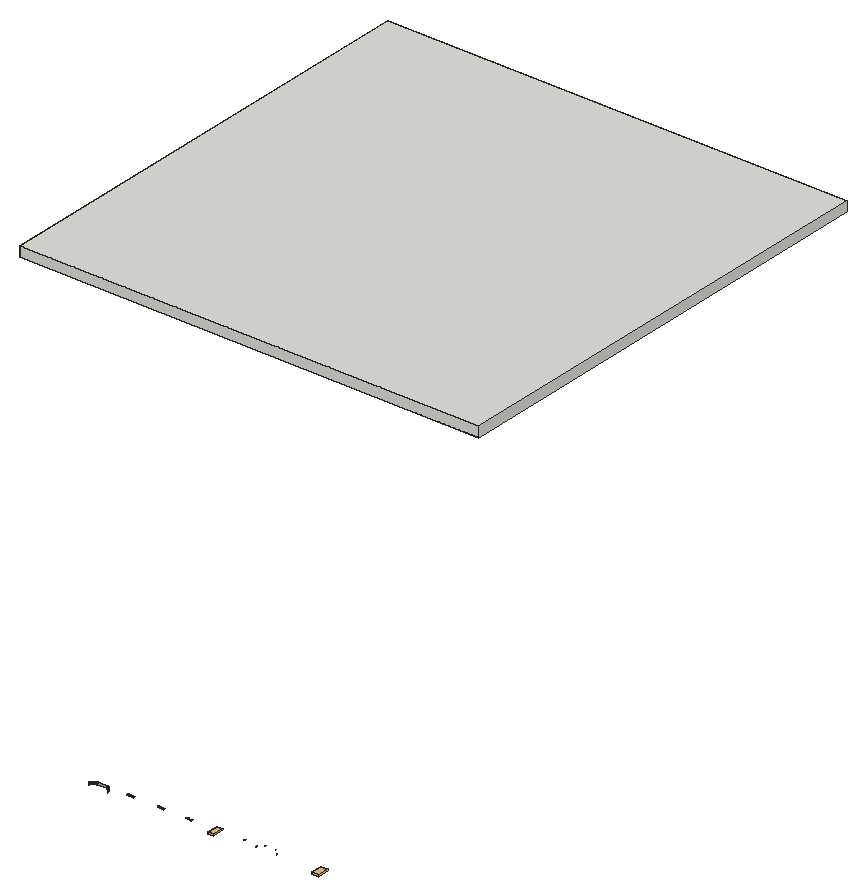
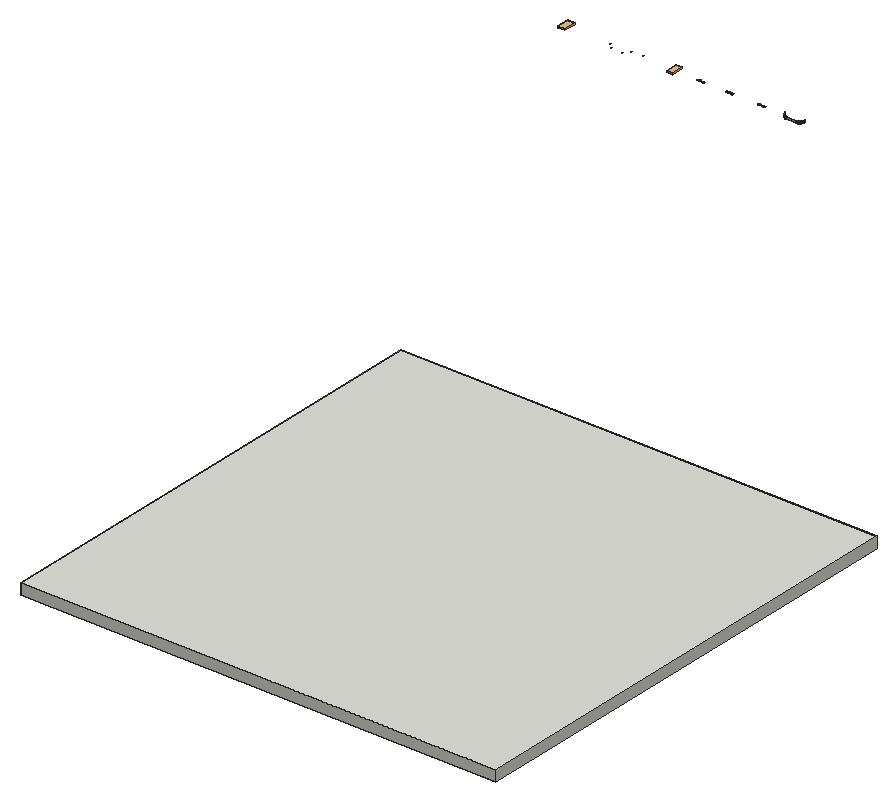
# SketchUp Ruby script. Lengths in inches.
U = 1.inch
M = Sketchup.active_model
def pt(a) = Geom::Point3d.new(a.map { |v| v * U })
def face(e, loops, mat)
  f = e.add_face(loops[0].map { |a| pt(a) })
  loops[1..].each { |l| e.add_face(l.map { |a| pt(a) }).erase! }
  f.material = f.back_material = mat if mat
  f
end
# faces: each face lists its corners as indices into pts; further lists are holes
def faces(e, pts, list, mat = nil) = list.each { |f| face(e, (f[0].is_a?(Array) ? f : [f]).map { |l| l.map { |i| pts[i] } }, mat) }
# xy, xz, yz: faces in a plane at the given z, y or x. An outline is a flat list of corners, or four numbers for a rectangle; further outlines are holes
def ring(l) = l.size == 4 ? [[l[0], l[1]], [l[2], l[1]], [l[2], l[3]], [l[0], l[3]]] : l.each_slice(2).to_a
def flat(e, list, mat, &to3) = list.each { |f| face(e, (f[0].is_a?(Array) ? f : [f]).map { |l| ring(l).map { |u, v| to3.(u, v) } }, mat) }
def xy(e, z, list, mat = nil) = flat(e, list, mat) { |x, y| [x, y, z] }
def xz(e, y, list, mat = nil) = flat(e, list, mat) { |x, z| [x, y, z] }
def yz(e, x, list, mat = nil) = flat(e, list, mat) { |y, z| [x, y, z] }
def lines(e, pts, list) = list.each { |a, b| e.add_line(pt(pts[a]), pt(pts[b])) }
# prism: a flat outline (further loops are holes) pulled along v
def prism(e, loops, v, mat = nil)
  f = face(e, loops, mat); d = Geom::Vector3d.new(v.map { |x| x * U })
  f.pushpull(f.normal.samedirection?(d) ? d.length : -d.length)
end
def box(e, o, s, mat = nil) = prism(e, [[o, [o[0] + s[0], o[1], o[2]], [o[0] + s[0], o[1] + s[1], o[2]], [o[0], o[1] + s[1], o[2]]]], [0, 0, s[2]], mat)
def at(x, y, z, deg = 0) = Geom::Transformation.translation(pt([x, y, z])) * Geom::Transformation.rotation(ORIGIN, Z_AXIS, deg.degrees)
def axes(o, x, y, z) = Geom::Transformation.new([*x, 0, *y, 0, *z, 0, *pt(o).to_a, 1])
def part(name) = M.definitions.add(name)
# library, detail: a bought-in or finely detailed component or shape, given as its bounding box
def library(name, o, s) = part(name).tap { |d| box(d.entities, o, s) }
def detail(e, o, s) = box(e.add_group.entities, o, s)
def put(e, d, t, mat = nil) = e.add_instance(d, t).tap { |i| i.material = mat if mat }
def group(e, t, mat = nil) = e.add_group.tap { |g| g.transformation = t; g.material = mat if mat }.entities
root = M.entities
M.materials.add("1").color = [0, 0, 0]
M.materials.add("21").color = [186, 186, 186]
M.materials.add("22").color = [12, 12, 12]
M.materials.add("23").color = [196, 196, 196]
M.materials.add("25").color = [154, 148, 138]
M.materials.add("26").color = [169, 186, 191]
M.materials.add("8").color = [50, 50, 50]
M.materials.add("[0132_LightGray]").color = [165, 152, 148]
c1 = library("Group4",[-46.72,-138.36,-0.02],[93.4,160.65,19.67])
c2 = library("Group40",[-41.15,-138.36,-0.05],[82.3,160.65,19.67])
c3 = library("om.cn_51995440",[-37.7,-5.67,0],[271.8,11.34,2])
c4 = library("om.cn_52",[-37.7,-5.67,0],[73.39,11.34,2])
xy(root,90.6622,[[287.484,13.1133,287.4883,13.1428,287.4929,13.1723],[287.484,13.1133,287.4929,13.1723,287.4979,13.2018],[287.484,13.1133,287.5144,13.2897,287.5204,13.3184]],"26")
xy(root,91.8361,[[298.2914,13.0775,298.2831,13.136,298.2737,13.194],[287.529,13.107,287.5378,13.165,287.5333,13.136],[287.5378,13.165,287.5478,13.223,287.5427,13.194],[298.2737,13.194,298.2685,13.223,298.2631,13.2518],[298.2631,13.2518,298.2574,13.2807,298.2516,13.3082],
  [289.8369,15.5804,289.8933,15.5919,289.8645,15.5862],[289.8933,15.5919,289.9511,15.6025,289.9222,15.5973],[295.8942,15.5973,295.8652,15.6025,295.8362,15.6073],[289.9511,15.6025,290.0677,15.6202,290.0091,15.6119],[295.8362,15.6073,295.8072,15.6119,295.7782,15.6161],
  [290.0091,15.6119,290.0677,15.6202,290.0382,15.6161],[295.7782,15.6161,295.7487,15.6202,295.7192,15.6239],[290.0677,15.6202,290.1267,15.6273,290.0972,15.6239],[290.0677,15.6202,290.1859,15.6333,290.1563,15.6305,290.1267,15.6273],[295.7192,15.6239,295.6896,15.6273,295.66,15.6305],
  [295.66,15.6305,295.6304,15.6333,295.6008,15.6359],[290.1859,15.6333,290.244,15.638,290.2155,15.6359]],"26")
xy(root,92.317,[[393.1555,13.5733,393.1532,13.6036,393.1505,13.6353],[381.6241,13.6036,381.6299,13.6669,381.6269,13.6353],[393.1505,13.6353,393.1475,13.6669,393.1441,13.6985,393.1364,13.7615],[381.6299,13.6669,381.6369,13.73,381.6332,13.6985],[393.1441,13.6985,393.1404,13.73,393.1364,13.7615],
  [381.6369,13.73,381.6452,13.793,381.6409,13.7615],[393.1364,13.7615,393.1276,13.824,393.1175,13.886],[393.1364,13.7615,393.1321,13.793,393.1276,13.824],[381.6452,13.793,381.6546,13.855,381.6498,13.824],[381.6546,13.855,381.6653,13.9169,381.6598,13.886],
  [393.1175,13.886,393.112,13.9169,393.1062,13.9477],[393.1062,13.9477,393.1001,13.9785,393.094,14.0079],[384.1094,16.434,384.1696,16.4462,384.1388,16.4401],[384.1696,16.4462,384.2314,16.4575,384.2005,16.452],[390.5769,16.452,390.546,16.4575,390.515,16.4627],
  [384.2314,16.4575,384.3558,16.4764,384.2933,16.4676],[390.515,16.4627,390.4841,16.4676,390.453,16.4721],[384.2933,16.4676,384.3558,16.4764,384.3243,16.4721],[390.453,16.4721,390.4216,16.4764,390.39,16.4804],[384.3558,16.4764,384.4189,16.4841,384.3873,16.4804],
  [384.3558,16.4764,384.4821,16.4905,384.4504,16.4874,384.4189,16.4841],[390.39,16.4804,390.3585,16.4841,390.3269,16.4874],[390.3269,16.4874,390.2953,16.4905,390.2637,16.4932],[384.4821,16.4905,384.544,16.4955,384.5137,16.4932]],"8")
xy(root,119.75,[[30.4587,526.4701,29.8602,526.5489,29.3025,526.7799,28.8235,527.1474,28.456,527.6263,28.225,528.184,28.1462,528.7826,28.225,529.3811,28.456,529.9388,28.8235,530.4177,29.3025,530.7852,29.8602,531.0163,30.4587,531.0951,31.0572,531.0163,31.615,530.7852,32.0939,530.4177,32.4614,529.9388,32.6924,529.3811,32.7712,528.7826,32.6924,528.184,32.4614,527.6263,32.0939,527.1474,31.615,526.7799,31.0572,526.5489],[73.515,526.4701,72.9164,526.5489,72.3587,526.7799,71.8798,527.1474,71.5123,527.6263,71.2812,528.184,71.2025,528.7826,71.2812,529.3811,71.5123,529.9388,71.8798,530.4177,72.3587,530.7852,72.9164,531.0163,73.515,531.0951,74.1135,531.0163,74.6712,530.7852,75.1501,530.4177,75.5176,529.9388,75.7487,529.3811,75.8275,528.7826,75.7487,528.184,75.5176,527.6263,75.1501,527.1474,74.6712,526.7799,74.1135,526.5489],[164.39,526.4701,163.7914,526.5489,163.2337,526.7799,162.7548,527.1474,162.3873,527.6263,162.1562,528.184,162.0775,528.7826,162.1562,529.3811,162.3873,529.9388,162.7548,530.4177,163.2337,530.7852,163.7914,531.0163,164.39,531.0951,164.9885,531.0163,165.5462,530.7852,166.0251,530.4177,166.3926,529.9388,166.6237,529.3811,166.7025,528.7826,166.6237,528.184,166.3926,527.6263,166.0251,527.1474,165.5462,526.7799,164.9885,526.5489],[209.8326,526.4701,209.2341,526.5489,208.6764,526.7799,208.1974,527.1474,207.8299,527.6263,207.5989,528.184,207.5201,528.7826,207.5989,529.3811,207.8299,529.9388,208.1974,530.4177,208.6764,530.7852,209.2341,531.0163,209.8326,531.0951,210.4311,531.0163,210.9889,530.7852,211.4678,530.4177,211.8353,529.9388,212.0663,529.3811,212.1451,528.7826,212.0663,528.184,211.8353,527.6263,211.4678,527.1474,210.9889,526.7799,210.4311,526.5489]])
xy(root,120,[[0,323.9222,0,583.2087,259.2865,583.2087,259.2865,323.9222,246.5495,323.9222,246.5495,570.4717,12.737,570.4717,12.737,323.9222],[12.737,546.4717,12.737,558.4717,246.5495,558.4717,246.5495,546.4717,217.8495,546.4717,217.8495,546.7717,217.5495,546.7717,217.5495,546.4717,188.8495,546.4717,188.8495,546.7717,188.5495,546.7717,188.5495,546.4717,159.8495,546.4717,159.8495,546.7717,159.5495,546.7717,159.5495,546.4717,123.8495,546.4717,123.8495,546.7717,123.5495,546.7717,123.5495,546.4717,94.8495,546.4717,94.8495,546.7717,94.5495,546.7717,94.5495,546.4717,65.8495,546.4717,65.8495,546.7717,65.5495,546.7717,65.5495,546.4717,36.8495,546.4717,36.8495,546.7717,36.5495,546.7717,36.5495,546.4717],[12.737,558.4717,246.5495,570.4717]])
xy(root,120,[[[12.737,323.9222,12.737,546.4717,36.5495,546.4717,36.5495,546.7717,36.8495,546.7717,36.8495,546.4717,65.5495,546.4717,65.5495,546.7717,65.8495,546.7717,65.8495,546.4717,94.5495,546.4717,94.5495,546.7717,94.8495,546.7717,94.8495,546.4717,123.5495,546.4717,123.5495,546.7717,123.8495,546.7717,123.8495,546.4717,159.5495,546.4717,159.5495,546.7717,159.8495,546.7717,159.8495,546.4717,188.5495,546.4717,188.5495,546.7717,188.8495,546.7717,188.8495,546.4717,217.5495,546.4717,217.5495,546.7717,217.8495,546.7717,217.8495,546.4717,246.5495,546.4717,246.5495,323.9222],[30.4587,526.4701,31.0572,526.5489,31.615,526.7799,32.0939,527.1474,32.4614,527.6263,32.6924,528.184,32.7712,528.7826,32.6924,529.3811,32.4614,529.9388,32.0939,530.4177,31.615,530.7852,31.0572,531.0163,30.4587,531.0951,29.8602,531.0163,29.3025,530.7852,28.8235,530.4177,28.456,529.9388,28.225,529.3811,28.1462,528.7826,28.225,528.184,28.456,527.6263,28.8235,527.1474,29.3025,526.7799,29.8602,526.5489],[73.515,526.4701,74.1135,526.5489,74.6712,526.7799,75.1501,527.1474,75.5176,527.6263,75.7487,528.184,75.8275,528.7826,75.7487,529.3811,75.5176,529.9388,75.1501,530.4177,74.6712,530.7852,74.1135,531.0163,73.515,531.0951,72.9164,531.0163,72.3587,530.7852,71.8798,530.4177,71.5123,529.9388,71.2812,529.3811,71.2025,528.7826,71.2812,528.184,71.5123,527.6263,71.8798,527.1474,72.3587,526.7799,72.9164,526.5489],[164.39,526.4701,164.9885,526.5489,165.5462,526.7799,166.0251,527.1474,166.3926,527.6263,166.6237,528.184,166.7025,528.7826,166.6237,529.3811,166.3926,529.9388,166.0251,530.4177,165.5462,530.7852,164.9885,531.0163,164.39,531.0951,163.7914,531.0163,163.2337,530.7852,162.7548,530.4177,162.3873,529.9388,162.1562,529.3811,162.0775,528.7826,162.1562,528.184,162.3873,527.6263,162.7548,527.1474,163.2337,526.7799,163.7914,526.5489],[209.8326,526.4701,210.4311,526.5489,210.9889,526.7799,211.4678,527.1474,211.8353,527.6263,212.0663,528.184,212.1451,528.7826,212.0663,529.3811,211.8353,529.9388,211.4678,530.4177,210.9889,530.7852,210.4311,531.0163,209.8326,531.0951,209.2341,531.0163,208.6764,530.7852,208.1974,530.4177,207.8299,529.9388,207.5989,529.3811,207.5201,528.7826,207.5989,528.184,207.8299,527.6263,208.1974,527.1474,208.6764,526.7799,209.2341,526.5489]]],"[0132_LightGray]")
xy(root,126,[[0,323.9222,259.2865,583.2087]])
xz(root,15.7279,[[290.4563,90.6622,295.3601,91.8361]],"26")
xz(root,323.9222,[[0,120,259.2865,126]])
xz(root,583.2087,[[0,120,259.2865,126]])
yz(root,0,[[323.9222,120,583.2087,126]])
yz(root,259.2865,[[323.9222,120,583.2087,126]])
p = [[287.4475,13.1185,90.6622],[287.4475,13.1185,91.8361],[287.4519,13.1484,91.8361],[287.4519,13.1484,90.6622],[287.4565,13.1782,91.8361],[287.4565,13.1782,90.6622],
  [298.3645,13.1484,90.6622],[298.3645,13.1484,91.8361],[298.3689,13.1185,91.8361],[298.3689,13.1185,90.6622],[298.3598,13.1782,90.6622],[298.3598,13.1782,91.8361],
  [287.4615,13.208,91.8361],[287.4615,13.208,90.6622],[287.4668,13.2378,91.8361],[287.4668,13.2378,90.6622],[287.4724,13.2675,91.8361],[287.4724,13.2675,90.6622],
  [298.3495,13.2378,90.6622],[298.3495,13.2378,91.8361],[298.3548,13.208,91.8361],[298.3548,13.208,90.6622],[298.3439,13.2675,90.6622],[298.3439,13.2675,91.8361],
  [287.4783,13.2971,91.8361],[287.4783,13.2971,90.6622],[287.4845,13.3267,91.8361],[287.4845,13.3267,90.6622],[287.5353,13.5297,91.8361],[287.5353,13.5297,90.6622],
  [298.3381,13.2971,90.6622],[298.3381,13.2971,91.8361],[298.3319,13.3267,90.6622],[298.3319,13.3267,91.8361],[298.281,13.5297,90.6622],[298.281,13.5297,91.8361],
  [287.5996,13.7271,91.8361],[287.5996,13.7271,90.6622],[298.2167,13.7271,90.6622],[298.2167,13.7271,91.8361],[287.6768,13.9184,91.8361],[287.6768,13.9184,90.6622],
  [298.1396,13.9184,90.6622],[298.1396,13.9184,91.8361],[287.7662,14.103,91.8361],[287.7662,14.103,90.6622],[298.0501,14.103,90.6622],[298.0501,14.103,91.8361],
  [287.8676,14.2804,91.8361],[287.8676,14.2804,90.6622],[297.9488,14.2804,90.6622],[297.9488,14.2804,91.8361],[287.9802,14.4501,91.8361],[287.9802,14.4501,90.6622],
  [297.8361,14.4501,90.6622],[297.8361,14.4501,91.8361],[288.1036,14.6115,91.8361],[288.1036,14.6115,90.6622],[297.7127,14.6115,90.6622],[297.7127,14.6115,91.8361],
  [288.2374,14.7643,91.8361],[288.2374,14.7643,90.6622],[297.579,14.7643,90.6622],[297.579,14.7643,91.8361],[288.3809,14.9078,91.8361],[288.3809,14.9078,90.6622],
  [297.4355,14.9078,90.6622],[297.4355,14.9078,91.8361],[288.5336,15.0415,91.8361],[288.5336,15.0415,90.6622],[297.2827,15.0415,90.6622],[297.2827,15.0415,91.8361],
  [288.6951,15.1649,91.8361],[288.6951,15.1649,90.6622],[297.1213,15.1649,90.6622],[297.1213,15.1649,91.8361],[288.8648,15.2776,91.8361],[288.8648,15.2776,90.6622],
  [296.9516,15.2776,90.6622],[296.9516,15.2776,91.8361],[289.0422,15.3789,91.8361],[289.0422,15.3789,90.6622],[296.7742,15.3789,90.6622],[296.7742,15.3789,91.8361],
  [289.2268,15.4684,91.8361],[289.2268,15.4684,90.6622],[296.5896,15.4684,90.6622],[296.5896,15.4684,91.8361],[289.418,15.5455,91.8361],[289.418,15.5455,90.6622],
  [289.6154,15.6098,91.8361],[289.6154,15.6098,90.6622],[296.2009,15.6098,90.6622],[296.2009,15.6098,91.8361],[296.3983,15.5455,91.8361],[296.3983,15.5455,90.6622],
  [289.8185,15.6607,91.8361],[289.8185,15.6607,90.6622],[295.9979,15.6607,90.6622],[295.9979,15.6607,91.8361],[289.848,15.6669,91.8361],[289.848,15.6669,90.6622],
  [289.8777,15.6727,91.8361],[289.8777,15.6727,90.6622],[289.9074,15.6783,91.8361],[289.9074,15.6783,90.6622],[289.9371,15.6836,91.8361],[289.9371,15.6836,90.6622],
  [289.9669,15.6886,91.8361],[289.9669,15.6886,90.6622],[289.9968,15.6933,91.8361],[289.9968,15.6933,90.6622],[290.0266,15.6977,91.8361],[290.0266,15.6977,90.6622],
  [290.0569,15.7018,91.8361],[290.0569,15.7018,90.6622],[290.0873,15.7056,91.8361],[290.0873,15.7056,90.6622],[290.1176,15.7092,91.8361],[290.1176,15.7092,90.6622],
  [290.148,15.7124,91.8361],[290.148,15.7124,90.6622],[290.1785,15.7153,91.8361],[290.1785,15.7153,90.6622],[290.2089,15.7179,91.8361],[290.2089,15.7179,90.6622],
  [290.2394,15.7202,91.8361],[290.2394,15.7202,90.6622],[290.4563,15.7279,91.8361],[290.4563,15.7279,90.6622],[295.3601,15.7279,90.6622],[295.3601,15.7279,91.8361],
  [295.5769,15.7202,91.8361],[295.5769,15.7202,90.6622],[295.6379,15.7153,90.6622],[295.6379,15.7153,91.8361],[295.6683,15.7124,91.8361],[295.6683,15.7124,90.6622],
  [295.6074,15.7179,90.6622],[295.6074,15.7179,91.8361],[295.7291,15.7056,90.6622],[295.7291,15.7056,91.8361],[295.7594,15.7018,91.8361],[295.7594,15.7018,90.6622],
  [295.6987,15.7092,90.6622],[295.6987,15.7092,91.8361],[295.8494,15.6886,90.6622],[295.8494,15.6886,91.8361],[295.8792,15.6836,91.8361],[295.8792,15.6836,90.6622],
  [295.8196,15.6933,90.6622],[295.8196,15.6933,91.8361],[295.7897,15.6977,90.6622],[295.7897,15.6977,91.8361],[295.9387,15.6727,90.6622],[295.9387,15.6727,91.8361],
  [295.9683,15.6669,91.8361],[295.9683,15.6669,90.6622],[295.909,15.6783,90.6622],[295.909,15.6783,91.8361],[29.8602,526.5489,120],[29.3025,526.7799,120],
  [29.3025,526.7799,119.75],[29.8602,526.5489,119.75],[30.4587,526.4701,120],[30.4587,526.4701,119.75],[31.0572,526.5489,120],[31.0572,526.5489,119.75],
  [31.615,526.7799,120],[31.615,526.7799,119.75],[72.9164,526.5489,120],[72.3587,526.7799,120],[72.3587,526.7799,119.75],[72.9164,526.5489,119.75],
  [73.515,526.4701,120],[73.515,526.4701,119.75],[74.1135,526.5489,120],[74.1135,526.5489,119.75],[74.6712,526.7799,120],[74.6712,526.7799,119.75],
  [163.7914,526.5489,120],[163.2337,526.7799,120],[163.2337,526.7799,119.75],[163.7914,526.5489,119.75],[164.39,526.4701,120],[164.39,526.4701,119.75],
  [164.9885,526.5489,120],[164.9885,526.5489,119.75],[165.5462,526.7799,120],[165.5462,526.7799,119.75],[209.2341,526.5489,120],[208.6764,526.7799,120],
  [208.6764,526.7799,119.75],[209.2341,526.5489,119.75],[209.8326,526.4701,120],[209.8326,526.4701,119.75],[210.4311,526.5489,120],[210.4311,526.5489,119.75],
  [210.9889,526.7799,120],[210.9889,526.7799,119.75],[28.8235,527.1474,120],[28.8235,527.1474,119.75],[32.0939,527.1474,120],[32.0939,527.1474,119.75],
  [71.8798,527.1474,120],[71.8798,527.1474,119.75],[75.1501,527.1474,120],[75.1501,527.1474,119.75],[162.7548,527.1474,120],[162.7548,527.1474,119.75],
  [166.0251,527.1474,120],[166.0251,527.1474,119.75],[208.1974,527.1474,120],[208.1974,527.1474,119.75],[211.4678,527.1474,120],[211.4678,527.1474,119.75],
  [28.456,527.6263,120],[28.456,527.6263,119.75],[32.4614,527.6263,120],[32.4614,527.6263,119.75],[71.5123,527.6263,120],[71.5123,527.6263,119.75],
  [75.5176,527.6263,120],[75.5176,527.6263,119.75],[162.3873,527.6263,120],[162.3873,527.6263,119.75],[166.3926,527.6263,120],[166.3926,527.6263,119.75],
  [207.8299,527.6263,120],[207.8299,527.6263,119.75],[211.8353,527.6263,120],[211.8353,527.6263,119.75],[28.225,528.184,120],[28.225,528.184,119.75],
  [32.6924,528.184,120],[32.6924,528.184,119.75],[71.2812,528.184,120],[71.2812,528.184,119.75],[75.7487,528.184,120],[75.7487,528.184,119.75],
  [162.1562,528.184,120],[162.1562,528.184,119.75],[166.6237,528.184,120],[166.6237,528.184,119.75],[207.5989,528.184,120],[207.5989,528.184,119.75],
  [212.0663,528.184,120],[212.0663,528.184,119.75],[28.1462,528.7826,120],[28.1462,528.7826,119.75],[32.7712,528.7826,120],[32.7712,528.7826,119.75],
  [71.2025,528.7826,120],[71.2025,528.7826,119.75],[75.8275,528.7826,120],[75.8275,528.7826,119.75],[162.0775,528.7826,120],[162.0775,528.7826,119.75],
  [166.7025,528.7826,120],[166.7025,528.7826,119.75],[207.5201,528.7826,120],[207.5201,528.7826,119.75],[212.1451,528.7826,120],[212.1451,528.7826,119.75],
  [28.225,529.3811,120],[28.225,529.3811,119.75],[32.6924,529.3811,120],[32.6924,529.3811,119.75],[71.2812,529.3811,120],[71.2812,529.3811,119.75],
  [75.7487,529.3811,120],[75.7487,529.3811,119.75],[162.1562,529.3811,120],[162.1562,529.3811,119.75],[166.6237,529.3811,120],[166.6237,529.3811,119.75],
  [207.5989,529.3811,120],[207.5989,529.3811,119.75],[212.0663,529.3811,120],[212.0663,529.3811,119.75],[28.456,529.9388,120],[28.456,529.9388,119.75],
  [32.4614,529.9388,120],[32.4614,529.9388,119.75],[71.5123,529.9388,120],[71.5123,529.9388,119.75],[75.5176,529.9388,120],[75.5176,529.9388,119.75],
  [162.3873,529.9388,120],[162.3873,529.9388,119.75],[166.3926,529.9388,120],[166.3926,529.9388,119.75],[207.8299,529.9388,120],[207.8299,529.9388,119.75],
  [211.8353,529.9388,120],[211.8353,529.9388,119.75],[28.8235,530.4177,120],[28.8235,530.4177,119.75],[32.0939,530.4177,120],[32.0939,530.4177,119.75],
  [71.8798,530.4177,120],[71.8798,530.4177,119.75],[75.1501,530.4177,120],[75.1501,530.4177,119.75],[162.7548,530.4177,120],[162.7548,530.4177,119.75],
  [166.0251,530.4177,120],[166.0251,530.4177,119.75],[208.1974,530.4177,120],[208.1974,530.4177,119.75],[211.4678,530.4177,120],[211.4678,530.4177,119.75],
  [29.3025,530.7852,120],[29.3025,530.7852,119.75],[31.615,530.7852,120],[31.615,530.7852,119.75],[72.3587,530.7852,120],[72.3587,530.7852,119.75],
  [74.6712,530.7852,120],[74.6712,530.7852,119.75],[163.2337,530.7852,120],[163.2337,530.7852,119.75],[165.5462,530.7852,120],[165.5462,530.7852,119.75],
  [208.6764,530.7852,120],[208.6764,530.7852,119.75],[210.9889,530.7852,120],[210.9889,530.7852,119.75],[29.8602,531.0163,120],[29.8602,531.0163,119.75],
  [31.0572,531.0163,120],[31.0572,531.0163,119.75],[72.9164,531.0163,120],[72.9164,531.0163,119.75],[74.1135,531.0163,120],[74.1135,531.0163,119.75],
  [163.7914,531.0163,120],[163.7914,531.0163,119.75],[164.9885,531.0163,120],[164.9885,531.0163,119.75],[209.2341,531.0163,120],[209.2341,531.0163,119.75],
  [210.4311,531.0163,120],[210.4311,531.0163,119.75],[30.4587,531.0951,120],[30.4587,531.0951,119.75],[73.515,531.0951,120],[73.515,531.0951,119.75],
  [164.39,531.0951,120],[164.39,531.0951,119.75],[209.8326,531.0951,120],[209.8326,531.0951,119.75]]
faces(root,p,[[0,1,2,3],[3,2,4,5],[6,7,8,9],[10,11,7,6],[5,4,12,13],[13,12,14,15],[15,14,16,17],[18,19,20,21],
  [22,23,19,18],[21,20,11,10],[17,16,24,25],[25,24,26,27],[27,26,28,29],[30,31,23,22],[32,33,31,30],[34,35,33,32],
  [29,28,36,37],[38,39,35,34],[37,36,40,41],[42,43,39,38],[41,40,44,45],[46,47,43,42],[45,44,48,49],[50,51,47,46],
  [49,48,52,53],[54,55,51,50],[53,52,56,57],[58,59,55,54],[57,56,60,61],[62,63,59,58],[61,60,64,65],[66,67,63,62],
  [65,64,68,69],[70,71,67,66],[69,68,72,73],[74,75,71,70],[73,72,76,77],[78,79,75,74],[77,76,80,81],[82,83,79,78],
  [81,80,84,85],[86,87,83,82],[85,84,88,89],[89,88,90,91],[92,93,94,95],[95,94,87,86],[91,90,96,97],[98,99,93,92],
  [97,96,100,101],[101,100,102,103],[103,102,104,105],[105,104,106,107],[107,106,108,109],[109,108,110,111],[111,110,112,113],[113,112,114,115],
  [115,114,116,117],[117,116,118,119],[119,118,120,121],[121,120,122,123],[123,122,124,125],[125,124,126,127],[127,126,128,129],[130,131,132,133],
  [134,135,136,137],[138,139,135,134],[133,132,139,138],[140,141,142,143],[144,145,141,140],[137,136,145,144],[146,147,148,149],[150,151,147,146],
  [152,153,151,150],[143,142,153,152],[154,155,156,157],[158,159,155,154],[149,148,159,158],[157,156,99,98]],"26")
faces(root,p,[[160,161,162,163],[164,160,163,165],[166,164,165,167],[168,166,167,169],[170,171,172,173],[174,170,173,175],[176,174,175,177],[178,176,177,179],
  [180,181,182,183],[184,180,183,185],[186,184,185,187],[188,186,187,189],[190,191,192,193],[194,190,193,195],[196,194,195,197],[198,196,197,199],
  [161,200,201,162],[202,168,169,203],[171,204,205,172],[206,178,179,207],[181,208,209,182],[210,188,189,211],[191,212,213,192],[214,198,199,215],
  [200,216,217,201],[218,202,203,219],[204,220,221,205],[222,206,207,223],[208,224,225,209],[226,210,211,227],[212,228,229,213],[230,214,215,231],
  [216,232,233,217],[234,218,219,235],[220,236,237,221],[238,222,223,239],[224,240,241,225],[242,226,227,243],[228,244,245,229],[246,230,231,247],
  [232,248,249,233],[250,234,235,251],[236,252,253,237],[254,238,239,255],[240,256,257,241],[258,242,243,259],[244,260,261,245],[262,246,247,263],
  [248,264,265,249],[266,250,251,267],[252,268,269,253],[270,254,255,271],[256,272,273,257],[274,258,259,275],[260,276,277,261],[278,262,263,279],
  [264,280,281,265],[282,266,267,283],[268,284,285,269],[286,270,271,287],[272,288,289,273],[290,274,275,291],[276,292,293,277],[294,278,279,295],
  [280,296,297,281],[298,282,283,299],[284,300,301,285],[302,286,287,303],[288,304,305,289],[306,290,291,307],[292,308,309,293],[310,294,295,311],
  [296,312,313,297],[314,298,299,315],[300,316,317,301],[318,302,303,319],[304,320,321,305],[322,306,307,323],[308,324,325,309],[326,310,311,327],
  [312,328,329,313],[330,314,315,331],[316,332,333,317],[334,318,319,335],[320,336,337,321],[338,322,323,339],[324,340,341,325],[342,326,327,343],
  [328,344,345,329],[344,330,331,345],[332,346,347,333],[346,334,335,347],[336,348,349,337],[348,338,339,349],[340,350,351,341],[350,342,343,351]])
put(root,c1,axes([417.67,15.4375,92.15],[0.0415,0,0],[0,0.03937,0],[0,0,0.0415]))
put(root,c2,axes([358.4,15.97,91.51],[0.03937,0,0],[0,0.03937,0],[0,0,0.03937]))
g1 = group(root,at(374.8,14.14,92.96))
xy(g1,0,[[-0.04,-0.32,-0.1,-0.3125,-0.16,-0.29,-0.22,-0.26,-0.26,-0.21,-0.29,-0.16,-0.3125,-0.1,-0.32,-0.03,-0.3125,0.03,-0.29,0.09,-0.26,0.15,-0.21,0.19,-0.16,0.22,-0.1,0.24,-0.03,0.25,0.03,0.24,0.09,0.22,0.15,0.1875,0.19,0.14,0.22,0.09,0.24,0.03,0.25,-0.04,0.24,-0.1,0.22,-0.16,0.1875,-0.22,0.14,-0.26,0.09,-0.29,0.03,-0.3125]],"1")
xy(g1,0.06,[[-0.04,-0.32,0.03,-0.3125,0.09,-0.29,0.14,-0.26,0.1875,-0.22,0.22,-0.16,0.24,-0.1,0.25,-0.04,0.24,0.03,0.22,0.09,0.19,0.14,0.15,0.1875,0.09,0.22,0.03,0.24,-0.03,0.25,-0.1,0.24,-0.16,0.22,-0.21,0.19,-0.26,0.15,-0.29,0.09,-0.3125,0.03,-0.32,-0.03,-0.3125,-0.1,-0.29,-0.16,-0.26,-0.21,-0.22,-0.26,-0.16,-0.29,-0.1,-0.3125]],"1")
p = [[-0.26,-0.21,0.06],[-0.26,-0.21,0],[-0.22,-0.26,0],[-0.22,-0.26,0.06],[-0.16,-0.29,0],[-0.16,-0.29,0.06],
  [-0.1,-0.3125,0],[-0.1,-0.3125,0.06],[-0.04,-0.32,0],[-0.04,-0.32,0.06],[0.03,-0.3125,0],[0.03,-0.3125,0.06],
  [0.09,-0.29,0],[0.09,-0.29,0.06],[0.14,-0.26,0],[0.14,-0.26,0.06],[0.1875,-0.22,0],[0.1875,-0.22,0.06],
  [-0.3125,-0.1,0.06],[-0.3125,-0.1,0],[-0.29,-0.16,0],[-0.29,-0.16,0.06],[0.22,-0.16,0],[0.22,-0.16,0.06],
  [0.24,-0.1,0],[0.24,-0.1,0.06],[-0.32,-0.03,0.06],[-0.32,-0.03,0],[0.25,-0.04,0],[0.25,-0.04,0.06],
  [-0.29,0.09,0.06],[-0.29,0.09,0],[-0.3125,0.03,0],[-0.3125,0.03,0.06],[0.24,0.03,0],[0.24,0.03,0.06],
  [0.22,0.09,0],[0.22,0.09,0.06],[-0.21,0.19,0.06],[-0.21,0.19,0],[-0.26,0.15,0],[-0.26,0.15,0.06],
  [0.19,0.14,0.06],[0.19,0.14,0],[0.15,0.1875,0],[0.15,0.1875,0.06],[-0.1,0.24,0.06],[-0.1,0.24,0],
  [-0.16,0.22,0],[-0.16,0.22,0.06],[-0.03,0.25,0.06],[-0.03,0.25,0],[0.09,0.22,0.06],[0.09,0.22,0],
  [0.03,0.24,0],[0.03,0.24,0.06]]
faces(g1,p,[[0,1,2,3],[3,2,4,5],[5,4,6,7],[7,6,8,9],[9,8,10,11],[11,10,12,13],[13,12,14,15],[15,14,16,17],
  [18,19,20,21],[21,20,1,0],[17,16,22,23],[23,22,24,25],[26,27,19,18],[25,24,28,29],[30,31,32,33],[33,32,27,26],
  [29,28,34,35],[35,34,36,37],[38,39,40,41],[41,40,31,30],[42,43,44,45],[37,36,43,42],[46,47,48,49],[49,48,39,38],
  [50,51,47,46],[52,53,54,55],[55,54,51,50],[45,44,53,52]],"1")
put(root,c3,axes([341.92,14.76,92.0625],[0.00983,0,0],[0,0.00983,0],[0,0,0.01124]),"22")
put(root,c4,axes([342.93,14.76,92.0625],[0.05136,0,0],[0,0.05136,0],[0,0,0.01475]),"21")
put(root,c3,axes([325.91,14.94,92.04],[0.00983,0,0],[0,0.00983,0],[0,0,0.03327]),"22")
put(root,c4,axes([326.92,14.94,92.04],[0.05136,0,0],[0,0.05136,0],[0,0,0.04368]),"23")
put(root,c3,axes([308.77,15.07,92.04],[0.00983,0,0],[0,0.00983,0],[0,0,0.03327]),"21")
put(root,c4,axes([309.77,15.07,92.04],[0.05136,0,0],[0,0.05136,0],[0,0,0.04368]),"25")
